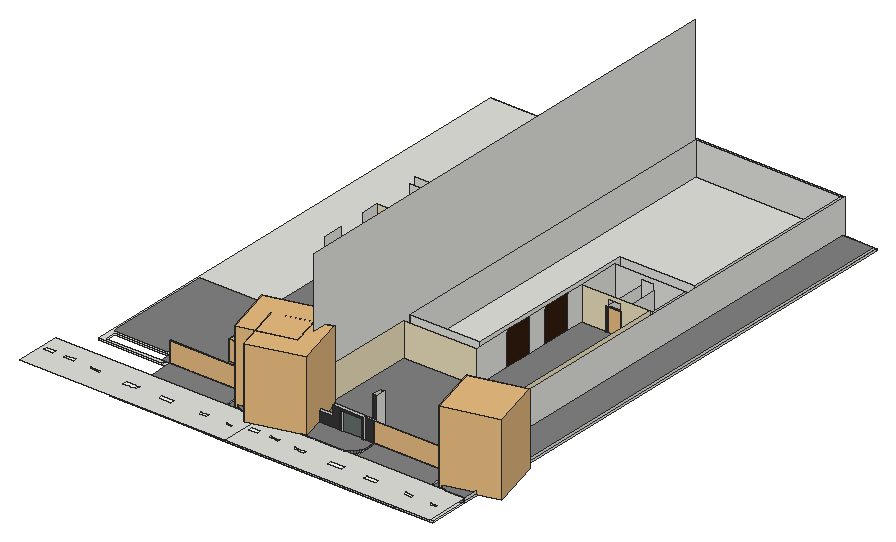
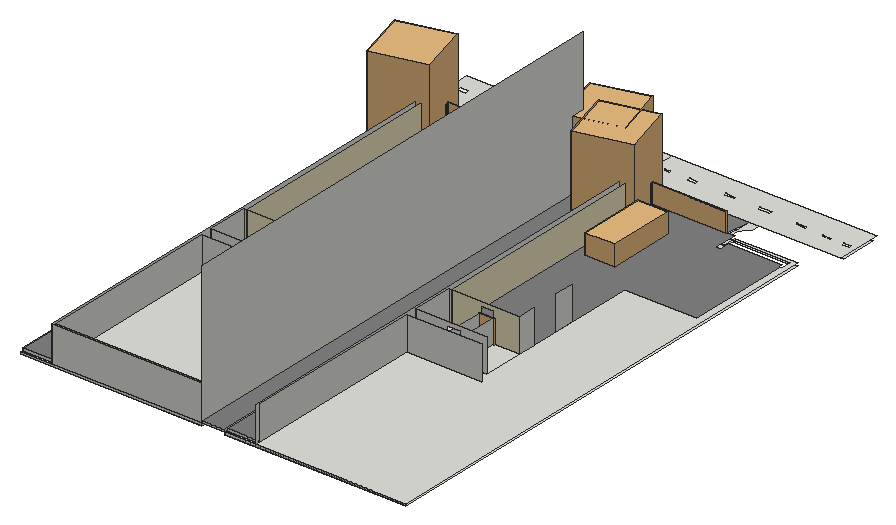
# SketchUp Ruby script. Lengths in inches.
U = 1.inch
M = Sketchup.active_model
def pt(a) = Geom::Point3d.new(a.map { |v| v * U })
def face(e, loops, mat)
  f = e.add_face(loops[0].map { |a| pt(a) })
  loops[1..].each { |l| e.add_face(l.map { |a| pt(a) }).erase! }
  f.material = f.back_material = mat if mat
  f
end
# faces: each face lists its corners as indices into pts; further lists are holes
def faces(e, pts, list, mat = nil) = list.each { |f| face(e, (f[0].is_a?(Array) ? f : [f]).map { |l| l.map { |i| pts[i] } }, mat) }
# xy, xz, yz: faces in a plane at the given z, y or x. An outline is a flat list of corners, or four numbers for a rectangle; further outlines are holes
def ring(l) = l.size == 4 ? [[l[0], l[1]], [l[2], l[1]], [l[2], l[3]], [l[0], l[3]]] : l.each_slice(2).to_a
def flat(e, list, mat, &to3) = list.each { |f| face(e, (f[0].is_a?(Array) ? f : [f]).map { |l| ring(l).map { |u, v| to3.(u, v) } }, mat) }
def xy(e, z, list, mat = nil) = flat(e, list, mat) { |x, y| [x, y, z] }
def xz(e, y, list, mat = nil) = flat(e, list, mat) { |x, z| [x, y, z] }
def yz(e, x, list, mat = nil) = flat(e, list, mat) { |y, z| [x, y, z] }
def lines(e, pts, list) = list.each { |a, b| e.add_line(pt(pts[a]), pt(pts[b])) }
# prism: a flat outline (further loops are holes) pulled along v
def prism(e, loops, v, mat = nil)
  f = face(e, loops, mat); d = Geom::Vector3d.new(v.map { |x| x * U })
  f.pushpull(f.normal.samedirection?(d) ? d.length : -d.length)
end
def box(e, o, s, mat = nil) = prism(e, [[o, [o[0] + s[0], o[1], o[2]], [o[0] + s[0], o[1] + s[1], o[2]], [o[0], o[1] + s[1], o[2]]]], [0, 0, s[2]], mat)
def at(x, y, z, deg = 0) = Geom::Transformation.translation(pt([x, y, z])) * Geom::Transformation.rotation(ORIGIN, Z_AXIS, deg.degrees)
def axes(o, x, y, z) = Geom::Transformation.new([*x, 0, *y, 0, *z, 0, *pt(o).to_a, 1])
def part(name) = M.definitions.add(name)
# library, detail: a bought-in or finely detailed component or shape, given as its bounding box
def library(name, o, s) = part(name).tap { |d| box(d.entities, o, s) }
def detail(e, o, s) = box(e.add_group.entities, o, s)
def put(e, d, t, mat = nil) = e.add_instance(d, t).tap { |i| i.material = mat if mat }
def group(e, t, mat = nil) = e.add_group.tap { |g| g.transformation = t; g.material = mat if mat }.entities
root = M.entities
M.materials.add("Color_000").color = [255, 255, 255]
M.materials.add("[Color D01]").color = [237, 225, 189]
M.materials.add("[Slate Light Tile]").color = [54, 54, 54]
M.materials.add("[Slate]").color = [102, 110, 108]
M.materials.add("[Tile Grey]").color = [130, 130, 130]
M.materials.add("[Wood Veneer 01]").color = [51, 28, 15]
c1 = part("Untitled (5)")
xy(c1.entities,0,[[[158.81,26.5625,306.06,993.3125],[226.57,518.17,239.57,583.92],[225.28,357.51,237.28,411.51],[222.61,182.28,236.36,226.53],[239.71,931.55,251.46,972.3],[233.64,703.93,242.14,755.18],[240.05,835.03,248.8,880.53],[222.04,66.5,231.29,100.5]]])
xy(c1.entities,0,[[222.04,66.5,231.29,100.5],[222.61,182.28,236.36,226.53],[225.28,357.51,237.28,411.51],[226.57,518.17,239.57,583.92],[233.64,703.93,242.14,755.18],
  [240.05,835.03,248.8,880.53],[239.71,931.55,251.46,972.3]],"Color_000")
c2 = library("Sliding Gate",[0,0,0],[194.88,4.13,70.58])
c3 = library("元件\#5",[-4.39,0,0],[5.37,35.83,90.55])
c4 = library("Group\#5",[0,0,0],[85.51,189.4,58.01])
c5 = part("2022 BMW i4")
put(c5.entities,c4,axes([0,0,0],[5,0,0],[0,5,0],[0,0,5]))
c6 = library("Palm tree",[-4.09,-4.52,0],[193.52,193.51,258.93])
c7 = part("Palm+Tree")
put(c7.entities,c6,at(25.51,-21.81,0,15))
xy(root,-6.875,[[1043.68,14.47,1043.68,164.29,1049.6,169.1875,1055.49,175.27,1060.67,181.96,1065.08,189.18,1068.68,196.84,1071.32,204.6,1071.32,246.64,1043.68,246.64,1043.68,294.84,1336.8,294.84,1336.8,14.47],[1336.8,14.47,1336.8,246.64,1339.28,246.64,1339.28,228.12,1341.81,219.11,1345.19,210.38,1349.375,202.01,1354.33,194.08,1360.01,186.64,1366.37,179.78,1373.35,173.54,1380.88,167.99,1388.91,163.18,1397.35,159.14,1467.125,159.14,1467.125,14.47],[1467.125,14.47,1467.125,159.14,1769.57,159.14,1776.64,163.79,1777.24,164.29,1777.24,14.47],[1777.24,14.47,1777.24,164.29,1783.16,169.1875,1789.05,175.27,1794.23,181.96,1798.65,189.18,1802.24,196.84,1804.89,204.6,1804.89,246.64,1777.24,246.64,1777.24,294.84,2070.36,294.84,2070.36,14.47],[2070.36,14.47,2070.36,246.64,2072.84,246.64,2072.84,228.12,2075.38,219.11,2078.75,210.38,2082.9375,202.01,2087.89,194.08,2093.57,186.64,2099.93,179.78,2106.91,173.54,2114.44,167.99,2122.47,163.18,2130.91,159.14,2200.6875,159.14,2200.6875,14.47],
  [1397.35,159.14,1388.91,163.18,1380.88,167.99,1373.35,173.54,1366.37,179.78,1360.01,186.64,1354.33,194.08,1349.375,202.01,1345.19,210.38,1341.81,219.11,1339.28,228.12,1339.28,246.64,1467.125,246.64,1467.125,159.14],[1467.125,159.14,1467.125,164.29,1777.24,164.29,1776.64,163.79,1769.57,159.14],[2130.91,159.14,2122.47,163.18,2114.44,167.99,2106.91,173.54,2099.93,179.78,2093.57,186.64,2087.89,194.08,2082.9375,202.01,2078.75,210.38,2075.38,219.11,2072.84,228.12,2072.84,246.64,2200.6875,246.64,2200.6875,159.14],[1467.125,164.29,1777.24,246.64],[1777.24,164.29,1777.24,246.64,1804.89,246.64,1804.89,204.6,1802.24,196.84,1798.65,189.18,1794.23,181.96,1789.05,175.27,1783.16,169.1875],
  [816.6875,246.64,816.6875,2003.89,1467.125,2003.89,1467.125,246.64,1336.8,246.64,1336.8,294.84,835.51,294.84,835.51,255.71,1043.68,255.71,1043.68,246.64],[1550.25,246.64,1550.25,2003.89,2200.6875,2003.89,2200.6875,246.64,2070.36,246.64,2070.36,294.84,1569.07,294.84,1569.07,255.71,1777.24,255.71,1777.24,246.64]])
xy(root,0,[[733.5625,14.47,1467.125,146.33],[1467.125,14.47,2200.6875,146.33],[1071.32,146.33,1336.8,204.6],[1336.8,146.33,1339.28,204.6],[1804.89,146.33,2070.36,204.6],
  [2070.36,146.33,2072.84,204.6],[1397.35,159.14,1467.125,159.14,1467.125,204.6,1348.08,204.6,1349.375,202.01,1354.33,194.08,1360.01,186.64,1366.37,179.78,1373.35,173.54,1380.88,167.99,1388.91,163.18],[1467.125,159.14,1769.57,159.14,1776.64,163.79,1777.24,164.29,1467.125,164.29],[2130.91,159.14,2200.6875,159.14,2200.6875,204.6,2081.64,204.6,2082.9375,202.01,2087.89,194.08,2093.57,186.64,2099.93,179.78,2106.91,173.54,2114.44,167.99,2122.47,163.18],[1467.125,164.29,1777.24,246.64],
  [1777.24,164.29,1783.16,169.1875,1789.05,175.27,1794.23,181.96,1798.65,189.18,1802.24,196.84,1804.89,204.6,1804.89,246.64,1777.24,246.64],[1071.32,204.6,1336.8,204.6,1336.8,246.64,1071.32,246.64,1073.1875,238.39,1074.14,229.98,1074.15,221.52,1073.24,213.11,1071.41,204.85],[1336.8,204.6,1339.28,204.6,1339.28,228.12,1337.6,237.32,1336.8,246.64],[1348.08,204.6,1467.125,204.6,1467.125,246.64,1339.28,246.64,1339.28,228.12,1341.81,219.11,1345.19,210.38],[1804.89,204.6,1804.97,204.85,1806.8,213.11,1807.72,221.52,1807.7,229.98,1806.75,238.39,1804.89,246.64],
  [1804.89,204.6,2070.36,204.6,2070.36,246.64,1804.89,246.64,1806.75,238.39,1807.7,229.98,1807.72,221.52,1806.8,213.11,1804.97,204.85],[2070.36,204.6,2072.84,204.6,2072.84,228.12,2071.16,237.32,2070.36,246.64],[2081.64,204.6,2200.6875,204.6,2200.6875,246.64,2072.84,246.64,2072.84,228.12,2075.38,219.11,2078.75,210.38],[1339.28,228.12,1339.28,246.64,1336.8,246.64,1337.6,237.32],[2072.84,228.12,2072.84,246.64,2070.36,246.64,2071.16,237.32],
  [816.6875,246.64,1043.68,246.64,1043.68,255.71,835.51,255.71,835.51,294.84,1336.8,294.84,1336.8,246.64,1355.5625,246.64,1355.5625,2003.89,816.6875,2003.89],[1071.32,246.64,1336.8,246.64,1336.8,294.84,1043.68,294.84,1043.68,255.71,1071.32,255.71],[1355.5625,246.64,1467.125,1994.39],[1467.125,246.64,1550.25,2003.89],[1550.25,246.64,1777.24,246.64,1777.24,255.71,1569.07,255.71,1569.07,294.84,2070.36,294.84,2070.36,246.64,2089.125,246.64,2089.125,2003.89,1550.25,2003.89],
  [1777.24,246.64,1804.89,255.71],[1804.89,246.64,2070.36,246.64,2070.36,294.84,1777.24,294.84,1777.24,255.71,1804.89,255.71],[2089.125,246.64,2200.6875,1994.39],[1355.5625,1994.39,1467.125,2003.89],[2089.125,1994.39,2200.6875,2003.89]])
xy(root,0,[[1339.28,146.33,1467.125,146.33,1467.125,159.14,1397.35,159.14,1388.91,163.18,1380.88,167.99,1373.35,173.54,1366.37,179.78,1360.01,186.64,1354.33,194.08,1349.375,202.01,1348.08,204.6,1339.28,204.6],[1467.125,146.33,1804.89,146.33,1804.89,204.6,1802.24,196.84,1798.65,189.18,1794.23,181.96,1789.05,175.27,1783.16,169.1875,1777.24,164.29,1776.64,163.79,1769.57,159.14,1467.125,159.14],[2072.84,146.33,2200.6875,146.33,2200.6875,159.14,2130.91,159.14,2122.47,163.18,2114.44,167.99,2106.91,173.54,2099.93,179.78,2093.57,186.64,2087.89,194.08,2082.9375,202.01,2081.64,204.6,2072.84,204.6],[1339.28,204.6,1348.08,204.6,1345.19,210.38,1341.81,219.11,1339.28,228.12],[2072.84,204.6,2081.64,204.6,2078.75,210.38,2075.38,219.11,2072.84,228.12]],"[Tile Grey]")
xy(root,8.6875,[[1558.89,714.9,1811.2,714.9,1811.2,1340.4,2080.49,1340.4,2080.49,1995.26,1558.89,1995.26],[1092.25,1150.15,1185.65,1298.96],[1233.65,1150.15,1346.93,1298.96],[1825.8125,1150.15,1919.21,1298.96],[1967.21,1150.15,2080.49,1298.96]])
xy(root,8.6875,[[1397.35,159.14,1467.125,159.14,1467.125,1994.39,1355.5625,1994.39,1355.5625,246.64,1336.8,246.64,1337.6,237.32,1339.28,228.12,1341.81,219.11,1345.19,210.38,1349.375,202.01,1354.33,194.08,1360.01,186.64,1366.37,179.78,1373.35,173.54,1380.88,167.99,1388.91,163.18],[1467.125,159.14,1769.57,159.14,1776.64,163.79,1783.16,169.1875,1789.05,175.27,1794.23,181.96,1798.65,189.18,1802.24,196.84,1804.97,204.85,1806.8,213.11,1807.72,221.52,1807.7,229.98,1806.75,238.39,1804.89,246.64,1770.98,246.64,1770.98,243.46,1763.07,243.46,1763.07,246.64,1691.68,246.64,1691.68,243.46,1682.97,243.46,1682.97,246.64,1550.25,246.64,1550.25,2003.89,1467.125,2003.89],[2130.91,159.14,2200.6875,159.14,2200.6875,1994.39,2089.125,1994.39,2089.125,246.64,2070.36,246.64,2071.16,237.32,2072.84,228.12,2075.38,219.11,2078.75,210.38,2082.9375,202.01,2087.89,194.08,2093.57,186.64,2099.93,179.78,2106.91,173.54,2114.44,167.99,2122.47,163.18],[1043.68,246.64,1336.8,246.64,1336.8,1150.15,1233.65,1150.15,1233.65,1298.96,1185.65,1298.96,1185.65,1150.15,1092.25,1150.15,1092.25,679.27,833.39,679.27,833.39,310.87,835.51,310.87,835.51,294.84,1028.12,294.84,1028.12,329.78,1043.68,329.78],[1777.24,246.64,2070.36,246.64,2070.36,1150.15,1967.21,1150.15,1967.21,1298.96,1919.21,1298.96,1919.21,1150.15,1825.8125,1150.15,1825.8125,679.27,1566.95,679.27,1566.95,310.87,1569.07,310.87,1569.07,294.84,1761.68,294.84,1761.68,329.78,1777.24,329.78]],"[Tile Grey]")
xz(root,14.47,[[1043.68,-6.875,1336.8,0],[1336.8,-6.875,1467.125,0],[1467.125,-6.875,1777.24,0],[1777.24,-6.875,2070.36,0],[2070.36,-6.875,2200.6875,0]])
xz(root,159.14,[[1397.35,-6.875,1467.125,0],[1467.125,-6.875,1769.57,0],[2130.91,-6.875,2200.6875,0]])
xz(root,159.14,[[1397.35,0,1467.125,8.6875],[1467.125,0,1769.57,8.6875],[2130.91,0,2200.6875,8.6875]],"[Tile Grey]")
xz(root,243.46,[[1682.97,8.6875,1691.68,8.6875,1691.68,74.24,1763.07,74.24,1763.07,8.6875,1770.98,8.6875,1770.98,79.95,1682.97,79.95]],"[Slate Light Tile]")
xz(root,246.64,[[1336.8,-6.875,1339.28,0],[1339.28,-6.875,1467.125,0],[1467.125,-6.875,1550.25,0],[1550.25,-6.875,1777.24,0],[1777.24,-6.875,1804.89,0],
  [2070.36,-6.875,2072.84,0],[2072.84,-6.875,2200.6875,0],[1071.32,0,1336.8,8.6875],[1336.8,0,1339.28,8.6875],[1777.24,0,1804.89,8.6875],
  [1804.89,0,2070.36,8.6875],[2070.36,0,2072.84,8.6875]])
xz(root,246.64,[[1336.8,8.6875,1355.5625,76.4375],[1550.25,8.6875,1682.97,8.6875,1682.97,79.95,1655.66,79.95,1655.66,44.76,1582.85,44.76,1582.85,79.95,1550.25,79.95],[1770.98,8.6875,1804.89,79.95],[2070.36,8.6875,2089.125,76.4375]],"[Slate Light Tile]")
xz(root,246.64,[[1691.68,8.6875,1763.07,74.24]],"[Slate]")
xz(root,255.71,[[1569.07,-6.875,1777.24,0],[1569.07,0,1569.07,79.95,1582.85,79.95,1582.85,44.76,1655.66,44.76,1655.66,79.95,1804.89,79.95,1804.89,0]])
xz(root,294.84,[[1043.68,-6.875,1336.8,0],[1569.07,-6.875,1761.68,0],[1761.68,-6.875,1777.24,0],[1777.24,-6.875,2070.36,0],[1569.07,0,1761.68,8.6875]])
xz(root,294.84,[[1761.68,0,1777.24,128.6875]],"[Slate Light Tile]")
xz(root,310.87,[[1566.95,8.6875,1569.07,128.6875]])
xz(root,329.78,[[1761.68,8.6875,1777.24,128.6875]])
xz(root,679.27,[[1566.95,8.6875,1825.8125,128.6875]],"[Color D01]")
xz(root,714.9,[[1558.89,8.6875,1811.2,128.6875]])
xz(root,1150.15,[[1336.8,8.6875,1346.93,128.6875],[2070.36,8.6875,2080.49,128.6875]])
xz(root,1150.15,[[1092.25,8.6875,1185.65,8.6875,1185.65,114.3125,1233.65,114.3125,1233.65,8.6875,1336.8,8.6875,1336.8,128.6875,1092.25,128.6875],[1825.8125,8.6875,1919.21,8.6875,1919.21,114.3125,1967.21,114.3125,1967.21,8.6875,2070.36,8.6875,2070.36,128.6875,1825.8125,128.6875]],"[Color D01]")
xz(root,1298.96,[[1092.25,8.6875,1092.25,128.6875,1346.93,128.6875,1346.93,8.6875,1233.65,8.6875,1233.65,114.3125,1185.65,114.3125,1185.65,8.6875],[1825.8125,8.6875,1825.8125,128.6875,2080.49,128.6875,2080.49,8.6875,1967.21,8.6875,1967.21,114.3125,1919.21,114.3125,1919.21,8.6875]])
xz(root,1340.4,[[1077.64,8.6875,1346.93,128.6875],[1811.2,8.6875,2080.49,128.6875]])
xz(root,1994.39,[[1355.5625,0,1467.125,8.6875],[2089.125,0,2200.6875,8.6875]])
xz(root,1995.26,[[1558.89,8.6875,2080.49,128.6875]])
xz(root,2003.89,[[816.6875,-6.875,1467.125,0],[1550.25,-6.875,2200.6875,0],[1467.125,0,1550.25,8.6875],[1550.25,0,2089.125,128.6875]])
yz(root,1092.25,[[914.71,8.6875,987.36,128.6875],[1088.15,8.6875,1150.15,128.6875]])
yz(root,1185.65,[[1150.15,8.6875,1298.96,91.5625]])
yz(root,1233.65,[[1150.15,8.6875,1298.96,91.5625]])
yz(root,1336.8,[[246.64,-6.875,286.21,0],[286.21,-6.875,294.84,0],[246.64,0,286.21,8.6875],[286.21,0,294.84,8.6875]])
yz(root,1336.8,[[316.26,8.6875,1150.15,128.6875]],"[Color D01]")
yz(root,1336.8,[[246.64,8.6875,286.21,76.4375],[286.21,8.6875,316.26,128.6875]],"[Slate Light Tile]")
yz(root,1339.28,[[228.12,-6.875,246.64,0],[146.33,0,228.12,0,228.12,7.08],[228.12,0,246.64,0,246.64,8.6875,228.12,7.08]])
yz(root,1346.93,[[1150.15,8.6875,1298.96,128.6875],[1340.4,8.6875,1995.26,128.6875]])
yz(root,1355.5625,[[1994.39,0,2003.89,0,2003.89,128.6875,286.21,128.6875,286.21,76.4375,246.64,76.4375,246.64,8.6875,1994.39,8.6875]])
yz(root,1467.125,[[14.47,-6.875,159.14,0],[159.14,-6.875,246.64,0],[246.64,-6.875,2003.89,0],[159.14,0,1994.39,8.6875],[1994.39,0,2003.89,8.6875]])
yz(root,1550.25,[[246.64,-6.875,2003.89,0],[246.64,8.6875,246.64,79.95,286.21,79.95,286.21,120.375,293.46,120.375,293.46,506.6875,2003.89,506.6875,2003.89,8.6875]])
yz(root,1558.89,[[714.9,8.6875,1995.26,128.6875]])
yz(root,1566.95,[[310.87,8.6875,679.27,128.6875]],"[Color D01]")
yz(root,1569.07,[[255.71,-6.875,286.21,0],[286.21,-6.875,294.84,0],[255.71,0,286.21,79.95]])
yz(root,1569.07,[[286.21,0,294.84,0,294.84,8.6875,310.87,8.6875,310.87,128.6875,286.21,128.6875]],"[Slate Light Tile]")
yz(root,1682.97,[[243.46,8.6875,246.64,79.95]])
yz(root,1691.68,[[243.46,8.6875,246.64,74.24]])
yz(root,1761.68,[[294.84,8.6875,329.78,128.6875]])
yz(root,1763.07,[[243.46,8.6875,246.64,74.24]])
yz(root,1770.98,[[243.46,8.6875,246.64,79.95]])
yz(root,1777.24,[[246.64,-6.875,255.71,0],[255.71,-6.875,294.84,0],[246.64,0,294.84,8.6875],[294.84,8.6875,329.78,128.6875]])
yz(root,1804.89,[[204.6,-6.875,246.64,0],[146.33,0,246.64,8.6875,246.64,0],[246.64,0,255.71,79.95]])
yz(root,1811.2,[[714.9,8.6875,1340.4,128.6875]])
yz(root,1825.8125,[[679.27,8.6875,818.04,128.6875],[914.71,8.6875,987.36,128.6875],[1088.15,8.6875,1150.15,128.6875],[1150.15,8.6875,1298.96,128.6875]])
yz(root,1825.8125,[[818.04,8.6875,914.71,128.6875],[987.36,8.6875,1088.15,128.6875]],"[Wood Veneer 01]")
yz(root,1919.21,[[1150.15,8.6875,1298.96,91.5625]])
yz(root,1967.21,[[1150.15,8.6875,1298.96,91.5625]])
yz(root,2070.36,[[246.64,-6.875,286.21,0],[286.21,-6.875,294.84,0],[246.64,0,286.21,8.6875],[286.21,0,294.84,8.6875]])
yz(root,2070.36,[[316.26,8.6875,1150.15,128.6875]],"[Color D01]")
yz(root,2070.36,[[246.64,8.6875,286.21,76.4375],[286.21,8.6875,316.26,128.6875]],"[Slate Light Tile]")
yz(root,2072.84,[[228.12,-6.875,246.64,0],[146.33,0,228.12,0,228.12,7.08],[228.12,0,246.64,0,246.64,8.6875,228.12,7.08]])
yz(root,2080.49,[[1150.15,8.6875,1298.96,128.6875],[1340.4,8.6875,1995.26,128.6875]])
yz(root,2089.125,[[1994.39,0,2003.89,0,2003.89,128.6875,286.21,128.6875,286.21,76.4375,246.64,76.4375,246.64,8.6875,1994.39,8.6875]])
yz(root,2200.6875,[[159.14,-6.875,246.64,0],[246.64,-6.875,2003.89,0],[159.14,0,1994.39,8.6875]])
p = [[1397.35,159.14,0],[1388.91,163.18,0],[1388.91,163.18,-6.875],[1397.35,159.14,-6.875],[1776.64,163.79,0],[1769.57,159.14,0],
  [1769.57,159.14,-6.875],[1776.64,163.79,-6.875],[2130.91,159.14,0],[2122.47,163.18,0],[2122.47,163.18,-6.875],[2130.91,159.14,-6.875],
  [1380.88,167.99,0],[1380.88,167.99,-6.875],[2114.44,167.99,0],[2114.44,167.99,-6.875],[1783.16,169.1875,0],[1777.24,164.29,0],
  [1777.24,164.29,-6.875],[1783.16,169.1875,-6.875],[1373.35,173.54,0],[1373.35,173.54,-6.875],[2106.91,173.54,0],[2106.91,173.54,-6.875],
  [1789.05,175.27,0],[1789.05,175.27,-6.875],[1366.37,179.78,0],[1366.37,179.78,-6.875],[2099.93,179.78,0],[2099.93,179.78,-6.875],
  [1794.23,181.96,0],[1794.23,181.96,-6.875],[1360.01,186.64,0],[1360.01,186.64,-6.875],[2093.57,186.64,0],[2093.57,186.64,-6.875],
  [1798.65,189.18,0],[1798.65,189.18,-6.875],[1354.33,194.08,0],[1354.33,194.08,-6.875],[2087.89,194.08,0],[2087.89,194.08,-6.875],
  [1802.24,196.84,0],[1802.24,196.84,-6.875],[1349.375,202.01,0],[1349.375,202.01,-6.875],[2082.9375,202.01,0],[2082.9375,202.01,-6.875],
  [1804.89,204.6,0],[1804.89,204.6,-6.875],[1348.08,204.6,0],[1345.19,210.38,0],[1345.19,210.38,-6.875],[2081.64,204.6,0],
  [2078.75,210.38,0],[2078.75,210.38,-6.875],[1341.81,219.11,0],[1341.81,219.11,-6.875],[2075.38,219.11,0],[2075.38,219.11,-6.875],
  [1339.28,228.12,0],[1339.28,228.12,-6.875],[2072.84,228.12,0],[2072.84,228.12,-6.875],[1071.32,246.64,8.6875],[1071.32,146.33,0],
  [1336.8,146.33,0],[1339.28,146.33,0],[1339.28,228.12,7.08],[1339.28,246.64,8.6875],[1336.8,246.64,8.6875],[1804.89,246.64,8.6875],
  [1804.89,146.33,0],[2070.36,146.33,0],[2072.84,146.33,0],[2072.84,228.12,7.08],[2072.84,246.64,8.6875],[2070.36,246.64,8.6875],
  [1397.35,159.14,8.6875],[1388.91,163.18,8.6875],[1776.64,163.79,8.6875],[1769.57,159.14,8.6875],[2130.91,159.14,8.6875],[2122.47,163.18,8.6875],
  [1380.88,167.99,8.6875],[2114.44,167.99,8.6875],[1783.16,169.1875,8.6875],[1373.35,173.54,8.6875],[2106.91,173.54,8.6875],[1789.05,175.27,8.6875],
  [1366.37,179.78,8.6875],[2099.93,179.78,8.6875],[1794.23,181.96,8.6875],[1360.01,186.64,8.6875],[2093.57,186.64,8.6875],[1798.65,189.18,8.6875],
  [1354.33,194.08,8.6875],[2087.89,194.08,8.6875],[1802.24,196.84,8.6875],[1349.375,202.01,8.6875],[2082.9375,202.01,8.6875],[1804.97,204.85,8.6875],
  [1804.97,204.85,0],[1345.19,210.38,8.6875],[2078.75,210.38,8.6875],[1806.8,213.11,8.6875],[1806.8,213.11,0],[1341.81,219.11,8.6875],
  [2075.38,219.11,8.6875],[1807.72,221.52,8.6875],[1807.72,221.52,0],[1339.28,228.12,8.6875],[2072.84,228.12,8.6875],[1807.7,229.98,8.6875],
  [1807.7,229.98,0],[1337.6,237.32,8.6875],[1337.6,237.32,0],[2071.16,237.32,8.6875],[2071.16,237.32,0],[1806.75,238.39,8.6875],
  [1806.75,238.39,0],[1336.8,246.64,0],[2070.36,246.64,0],[1804.89,246.64,0]]
faces(root,p,[[0,1,2,3],[4,5,6,7],[8,9,10,11],[1,12,13,2],[9,14,15,10],[16,17,4,7,18,19],[12,20,21,13],[14,22,23,15],
  [24,16,19,25],[20,26,27,21],[22,28,29,23],[30,24,25,31],[26,32,33,27],[28,34,35,29],[36,30,31,37],[32,38,39,33],
  [34,40,41,35],[42,36,37,43],[38,44,45,39],[40,46,47,41],[48,42,43,49],[50,51,52,45,44],[53,54,55,47,46],[51,56,57,52],
  [54,58,59,55],[56,60,61,57],[58,62,63,59]])
faces(root,p,[[64,65,66,67,68,69,70],[71,72,73,74,75,76,77],[78,79,1,0],[80,81,5,4],[82,83,9,8],[79,84,12,1],[83,85,14,9],[86,80,4,17,16],
  [84,87,20,12],[85,88,22,14],[89,86,16,24],[87,90,26,20],[88,91,28,22],[92,89,24,30],[90,93,32,26],[91,94,34,28],
  [95,92,30,36],[93,96,38,32],[94,97,40,34],[98,95,36,42],[96,99,44,38],[97,100,46,40],[101,98,42,48,102],[99,103,51,50,44],
  [100,104,54,53,46],[105,101,102,106],[103,107,56,51],[104,108,58,54],[109,105,106,110],[107,111,68,60,56],[108,112,75,62,58],[113,109,110,114],
  [111,115,116,60,68],[112,117,118,62,75],[119,113,114,120],[115,70,121,116],[117,77,122,118],[71,119,120,123]],"[Tile Grey]")
put(root,c1,axes([1487.28,-171.64,8.6875],[0,1.08078,0],[-0.75879,0,0],[0,0,1]))
put(root,c2,axes([1071.32,246.64,8.6875],[1.37,0,0],[0,1,0],[0,0,1]))
put(root,c3,axes([1181.44,1151.01,-17.4375],[0,-0.89,0],[1.45734,0,0],[0,0,1.20374]))
put(root,c5,axes([1195.82,357.5625,8.6875],[0.25,0,0],[0,0.25,0],[0,0,0.25]))
put(root,c7,at(1336.8,204.6,0))
put(root,c7,at(1419.1875,141.91,0))
put(root,c1,axes([2220.84,-171.64,8.6875],[0,1.08078,0],[-0.75879,0,0],[0,0,1]))
put(root,c2,axes([1804.89,246.64,8.6875],[1.37,0,0],[0,1,0],[0,0,1]))
put(root,c3,axes([1915,1151.01,-17.4375],[0,-0.89,0],[1.45734,0,0],[0,0,1.20374]))
put(root,c7,at(2070.36,204.6,0))
